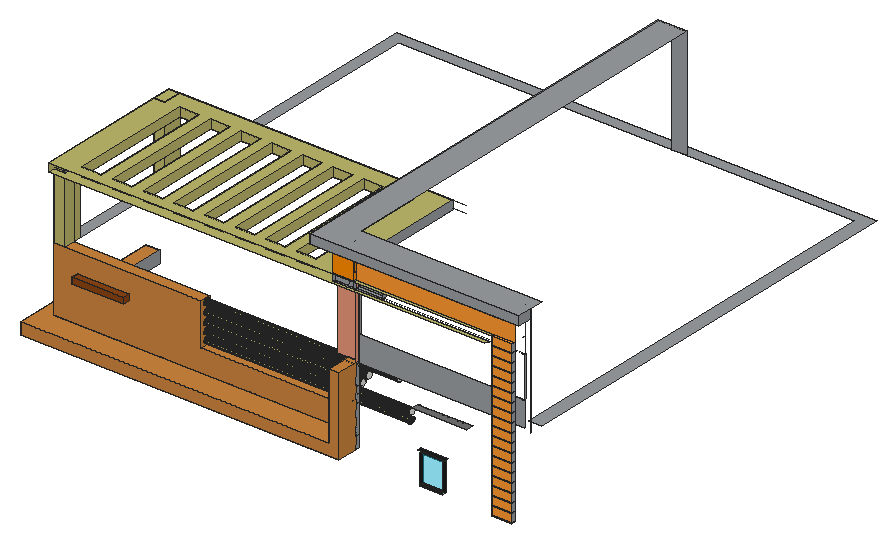
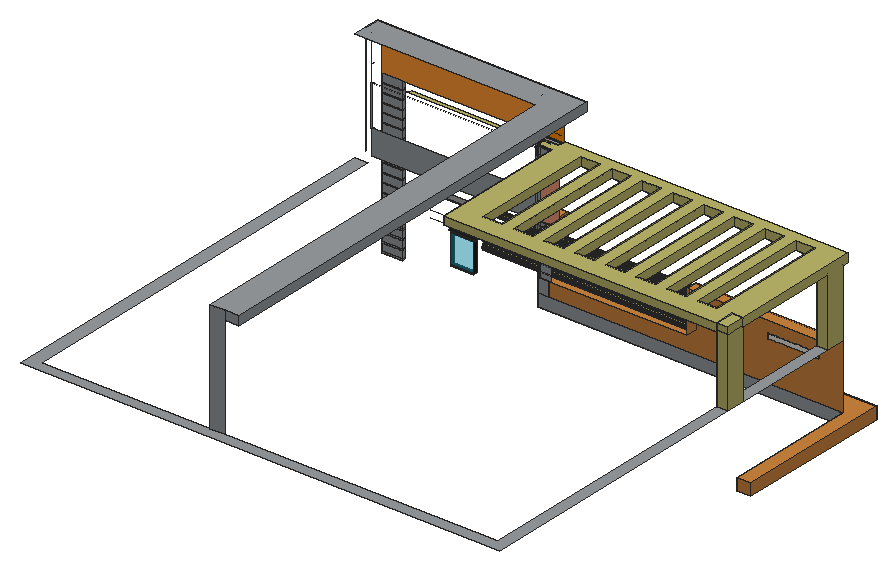
# SketchUp Ruby script. Lengths in inches.
U = 1.inch
M = Sketchup.active_model
def pt(a) = Geom::Point3d.new(a.map { |v| v * U })
def face(e, loops, mat)
  f = e.add_face(loops[0].map { |a| pt(a) })
  loops[1..].each { |l| e.add_face(l.map { |a| pt(a) }).erase! }
  f.material = f.back_material = mat if mat
  f
end
# faces: each face lists its corners as indices into pts; further lists are holes
def faces(e, pts, list, mat = nil) = list.each { |f| face(e, (f[0].is_a?(Array) ? f : [f]).map { |l| l.map { |i| pts[i] } }, mat) }
# xy, xz, yz: faces in a plane at the given z, y or x. An outline is a flat list of corners, or four numbers for a rectangle; further outlines are holes
def ring(l) = l.size == 4 ? [[l[0], l[1]], [l[2], l[1]], [l[2], l[3]], [l[0], l[3]]] : l.each_slice(2).to_a
def flat(e, list, mat, &to3) = list.each { |f| face(e, (f[0].is_a?(Array) ? f : [f]).map { |l| ring(l).map { |u, v| to3.(u, v) } }, mat) }
def xy(e, z, list, mat = nil) = flat(e, list, mat) { |x, y| [x, y, z] }
def xz(e, y, list, mat = nil) = flat(e, list, mat) { |x, z| [x, y, z] }
def yz(e, x, list, mat = nil) = flat(e, list, mat) { |y, z| [x, y, z] }
def lines(e, pts, list) = list.each { |a, b| e.add_line(pt(pts[a]), pt(pts[b])) }
# prism: a flat outline (further loops are holes) pulled along v
def prism(e, loops, v, mat = nil)
  f = face(e, loops, mat); d = Geom::Vector3d.new(v.map { |x| x * U })
  f.pushpull(f.normal.samedirection?(d) ? d.length : -d.length)
end
def box(e, o, s, mat = nil) = prism(e, [[o, [o[0] + s[0], o[1], o[2]], [o[0] + s[0], o[1] + s[1], o[2]], [o[0], o[1] + s[1], o[2]]]], [0, 0, s[2]], mat)
def at(x, y, z, deg = 0) = Geom::Transformation.translation(pt([x, y, z])) * Geom::Transformation.rotation(ORIGIN, Z_AXIS, deg.degrees)
def axes(o, x, y, z) = Geom::Transformation.new([*x, 0, *y, 0, *z, 0, *pt(o).to_a, 1])
def part(name) = M.definitions.add(name)
# library, detail: a bought-in or finely detailed component or shape, given as its bounding box
def library(name, o, s) = part(name).tap { |d| box(d.entities, o, s) }
def detail(e, o, s) = box(e.add_group.entities, o, s)
def put(e, d, t, mat = nil) = e.add_instance(d, t).tap { |i| i.material = mat if mat }
def group(e, t, mat = nil) = e.add_group.tap { |g| g.transformation = t; g.material = mat if mat }.entities
root = M.entities
M.materials.add("[0014_DarkSalmon]").color = [233, 150, 122]
M.materials.add("[0039_DarkOrange]").color = [255, 140, 0]
M.materials.add("[0040_Peru]").color = [205, 133, 63]
M.materials.add("[0043_SaddleBrown]").color = [139, 69, 19]
M.materials.add("[0057_DarkKhaki]").color = [189, 183, 107]
M.materials.add("[Color C04]").color = [255, 153, 50]
M.materials.add("[Color M05]").color = [114, 114, 114]
M.materials.add("[Color M08]").color = [30, 30, 30]
M.materials.add("[Metal Rough]").color = [153, 157, 160]
M.materials.add("[Translucent Glass Tinted]").color = [8, 201, 241]
M.materials["[Translucent Glass Tinted]"].alpha = 0.48
xy(root,144.5,[[415.14,37.17,432.3,40.17]],"[Color C04]")
xy(root,145.41,[[415.14,37.17,432.3,40.17]],"[Color C04]")
xy(root,150.37,[[359.96,31.17,379.6,34.17]],"[Color M08]")
xy(root,151.38,[[359.96,31.17,379.6,34.17]],"[Color M08]")
xy(root,152,[[415.14,37.17,432.3,40.17]],"[Color C04]")
xy(root,152.08,[[31.17,22.73,31.17,154.25,43.17,154.25,43.17,40.17,298.9,40.17,298.9,22.73]],"[0040_Peru]")
xy(root,152.08,[[43.17,40.17,298.9,40.42],[43.17,40.42,298.9,43.17]],"[Metal Rough]")
xy(root,152.91,[[415.14,37.17,432.3,40.17]],"[Color C04]")
xy(root,159.5,[[415.14,37.17,432.3,40.17]],"[Color C04]")
xy(root,160.41,[[415.14,37.17,432.3,40.17]],"[Color C04]")
xy(root,162,[[31.17,22.73,290.16,22.73,290.16,43.17,43.17,43.17,43.17,154.25,31.17,154.25]],"[0040_Peru]")
xy(root,167,[[415.14,37.17,432.3,40.17]],"[Color C04]")
xy(root,167.91,[[415.14,37.17,432.3,40.17]],"[Color C04]")
xy(root,174.5,[[415.14,37.17,432.3,40.17]],"[Metal Rough]")
xy(root,174.87,[[359.96,31.17,379.6,34.17]],"[Color M08]")
xy(root,175.41,[[415.14,37.17,432.3,40.17]],"[Color C04]")
xy(root,176.58,[[358.25,31.17,381.3125,34.17]],"[Color M08]")
xy(root,180.82,[[166.66,43.17,290.16,43.17,290.16,51.85,281.37,51.85,281.37,52.17,166.66,52.17]],"[0040_Peru]")
xy(root,180.82,[[281.37,51.85,290.16,52.17]],"[Metal Rough]")
xy(root,182,[[415.14,37.17,432.3,40.17]],"[Metal Rough]")
xy(root,182.91,[[415.14,37.17,432.3,40.17]],"[Color C04]")
xy(root,189.5,[[415.14,37.17,432.3,40.17]],"[Color C04]")
xy(root,190.41,[[415.14,37.17,432.3,40.17]],"[Color C04]")
xy(root,195.12,[[63.06,37.17,106.31,43.17]],"[0043_SaddleBrown]")
xy(root,197,[[415.14,37.17,432.3,40.17]],"[Color C04]")
xy(root,197.91,[[415.14,37.17,432.3,40.17]],"[Color C04]")
xy(root,200.18,[[63.06,37.17,106.31,43.17]],"[0043_SaddleBrown]")
xy(root,204.05,[[350.73,34.17,396.98,40.17]],"[Color M05]")
xy(root,204.05,[[350.73,40.17,389.11,40.42]],"[Metal Rough]")
xy(root,204.5,[[415.14,37.17,432.3,40.17]],"[Color C04]")
xy(root,205.41,[[415.14,37.17,432.3,40.17]],"[Color C04]")
xy(root,212,[[415.14,37.17,432.3,40.17]],"[Color C04]")
xy(root,212.91,[[415.14,37.17,432.3,40.17]],"[Color C04]")
xy(root,216.1875,[[52.23,43.17,166.66,52.17]],"[0040_Peru]")
xy(root,216.1875,[[43.17,43.17,43.17,58.8,52.17,58.8,52.17,52.17,52.23,52.17,52.23,43.17],[290.16,43.17,290.35,51.85],[290.16,51.85,293.27,52.17],[434.73,52.17,445.6,52.17,445.6,403.17,43.17,403.17,43.17,163.42,52.17,163.42,52.17,394.17,434.73,394.17],[52.17,52.17,52.23,58.8],
  [43.17,58.8,52.17,147.79],[43.17,147.79,52.17,163.42],[52.17,147.79,52.23,156.79]],"[Metal Rough]")
xy(root,217.4375,[[290.16,22.73,298.9,43.17]],"[0040_Peru]")
xy(root,217.4375,[[281.37,43.17,290.16,51.85],[290.16,43.17,290.35,51.85]],"[Metal Rough]")
xy(root,219.5,[[415.14,37.17,432.3,40.17]],"[Color C04]")
xy(root,220.41,[[415.14,37.17,432.3,40.17]],"[Color C04]")
xy(root,227,[[415.14,37.17,432.3,40.17]],"[Color C04]")
xy(root,227.91,[[415.14,37.17,432.3,40.17]],"[Color C04]")
xy(root,234.5,[[415.14,37.17,432.3,40.17]],"[Color C04]")
xy(root,235.41,[[415.14,37.17,432.3,40.17]],"[Color C04]")
xy(root,237.37,[[298.9,43.17,438.67,43.29]],"[Metal Rough]")
xy(root,242,[[415.14,37.17,432.3,40.17]],"[Color C04]")
xy(root,242.91,[[415.14,37.17,432.3,40.17]],"[Metal Rough]")
xy(root,249.5,[[415.14,37.17,432.3,40.17]],"[Color C04]")
xy(root,250.41,[[415.14,37.17,432.3,40.17]],"[Color C04]")
xy(root,257,[[415.14,37.17,432.3,40.17]],"[Color C04]")
xy(root,257.91,[[415.14,37.17,432.3,40.17]],"[Metal Rough]")
xy(root,264.5,[[415.14,37.17,432.3,40.17]],"[Color C04]")
xy(root,265.41,[[415.14,37.17,432.3,40.17]],"[Metal Rough]")
xy(root,265.6875,[[290.16,51.54,293.27,51.85]],"[Metal Rough]")
xy(root,271.4375,[[298.9,43.1,438.67,43.29]],"[Metal Rough]")
xy(root,272,[[415.14,37.17,432.3,40.17]],"[Color C04]")
xy(root,272.375,[[[43.17,37.17,43.17,43.17,52.23,43.17,52.23,52.17,52.17,52.17,52.17,58.8,43.17,58.8,43.17,147.79,52.17,147.79,52.17,163.42,281.37,163.42,281.37,50.92,293.27,50.92,293.27,43.17,281.37,43.17,281.37,40.17,411.24,40.17,409.48,37.17],[64.28,46.19,80.34,148.82],[90.03,46.19,106.09,148.82],[115.78,46.19,131.84,148.82],[141.53,46.19,157.59,148.82],[167.28,46.19,183.34,148.82],[193.03,46.19,209.09,148.82],[218.78,46.19,234.84,148.82],[244.53,46.19,260.59,148.82]]],"[0057_DarkKhaki]")
xy(root,272.91,[[415.14,37.17,432.3,40.17]],"[Metal Rough]")
xy(root,273.5,[[43.17,147.79,52.17,163.42]])
xy(root,273.5,[[293.27,38.17,298.9,38.17,298.9,40.17,281.37,40.17,281.37,38.42,293.27,38.42],[281.37,40.17,321.39,43.17],[51.48,43.17,52.17,52.17],[52.17,43.17,52.23,52.17]],"[Metal Rough]")
xy(root,279.5,[[[43.17,37.17,415.14,37.17,415.14,40.17,298.9,40.17,298.9,38.48,281.37,38.48,281.37,43.17,293.27,43.17,293.27,50.92,281.37,50.92,281.37,163.42,52.17,163.42,52.17,147.79,43.17,147.79],[64.28,46.19,80.34,148.82],[90.03,46.19,106.09,148.82],[115.78,46.19,131.84,148.82],[141.53,46.19,157.59,148.82],[167.28,46.19,183.34,148.82],[193.03,46.19,209.09,148.82],[218.78,46.19,234.84,148.82],[244.53,46.19,260.59,148.82]],[43.17,147.79,52.17,163.42]],"[0057_DarkKhaki]")
xy(root,279.5,[[415.14,37.17,432.3,40.17]],"[Color C04]")
xy(root,279.5,[[281.37,38.48,293.27,40.17],[293.27,38.48,298.9,40.17],[281.37,40.17,293.27,43.17],[293.27,40.17,298.9,43.17],[298.9,40.17,321.39,43.17],
  [281.37,50.92,293.27,51.54],[281.37,51.54,293.27,52.17]],"[Metal Rough]")
xy(root,301.86,[[281.37,38.48,298.9,38.54],[281.37,38.54,298.9,40.17]])
xy(root,301.86,[[269.68,28.17,269.68,394.17,281.37,394.17,281.37,38.48,298.9,38.48,298.9,40.17,432.3,40.17,428.02,28.17]],"[Color C04]")
xy(root,301.86,[[428.02,28.17,445.6,28.17,445.6,40.17,432.3,40.17]],"[Metal Rough]")
xy(root,309.37,[[269.68,28.17,445.6,28.17,445.6,52.17,293.27,52.17,293.27,394.17,269.68,394.17]],"[Metal Rough]")
xz(root,22.73,[[31.17,152.08,298.9,152.08,298.9,217.4375,290.16,217.4375,290.16,162,31.17,162]],"[0040_Peru]")
xz(root,28.17,[[269.68,301.86,445.6,309.37]],"[Metal Rough]")
xz(root,31.17,[[359.96,150.37,379.6,151.38]],"[Color M08]")
xz(root,34.17,[[359.96,150.37,379.6,151.38]])
xz(root,34.17,[[359.96,151.38,379.6,174.87]],"[Translucent Glass Tinted]")
xz(root,37.17,[[63.06,195.12,106.31,200.18]],"[0043_SaddleBrown]")
xz(root,37.17,[[415.14,145.41,432.3,152],[415.14,152.91,432.3,159.5],[415.14,160.41,432.3,167],[415.14,167.91,432.3,174.5],[415.14,175.41,432.3,182],
  [415.14,182.91,432.3,189.5],[415.14,190.41,432.3,197],[415.14,197.91,432.3,204.5],[415.14,205.41,432.3,212],[415.14,212.91,432.3,219.5],
  [415.14,220.41,432.3,227],[415.14,227.91,432.3,234.5],[415.14,235.41,432.3,242],[415.14,242.91,432.3,249.5],[415.14,250.41,432.3,257],
  [415.14,257.91,432.3,264.5],[415.14,265.41,432.3,272],[415.14,272.91,432.3,279.5]],"[Color C04]")
xz(root,38.48,[[281.37,279.5,298.9,301.86]],"[0039_DarkOrange]")
xz(root,40.17,[[415.14,189.5,432.3,190.41],[415.14,197,432.3,197.91],[415.14,204.5,432.3,205.41],[415.14,212,432.3,212.91],[415.14,219.5,432.3,220.41],
  [415.14,227,432.3,227.91],[415.14,234.5,432.3,235.41],[415.14,249.5,432.3,250.41],[415.14,257,432.3,257.91],[415.14,264.5,432.3,265.41],
  [415.14,272,432.3,272.91],[298.9,279.5,432.3,301.86]],"[Color C04]")
xz(root,40.17,[[415.14,144.5,432.3,145.41],[415.14,145.41,432.3,152],[415.14,152,432.3,152.91],[415.14,152.91,432.3,159.5],[415.14,159.5,432.3,160.41],
  [415.14,160.41,432.3,167],[415.14,167,432.3,167.91],[415.14,167.91,432.3,174.5],[415.14,174.5,432.3,175.41],[415.14,175.41,432.3,182],
  [415.14,182,432.3,182.91],[415.14,182.91,432.3,189.5],[415.14,190.41,432.3,197],[415.14,197.91,432.3,204.5],[415.14,205.41,432.3,212],
  [415.14,212.91,432.3,219.5],[415.14,220.41,432.3,227],[415.14,227.91,432.3,234.5],[415.14,235.41,432.3,242],[415.14,242,432.3,242.91],
  [415.14,242.91,432.3,249.5],[415.14,250.41,432.3,257],[415.14,257.91,432.3,264.5],[415.14,265.41,432.3,272],[281.37,272.375,293.27,273.5],
  [293.27,272.375,298.9,273.5],[298.9,272.375,321.39,273.5],[415.14,272.91,432.3,279.5],[281.37,273.5,293.27,279.5],[293.27,273.5,298.9,279.5]],"[Metal Rough]")
xz(root,43.17,[[63.06,195.12,106.31,200.18]])
xz(root,43.17,[[281.37,217.4375,298.9,217.4375,298.9,273.5,293.27,273.5,293.27,272.375,281.37,272.375]],"[0014_DarkSalmon]")
xz(root,43.17,[[[43.17,162,290.16,162,290.16,180.82,166.66,180.82,166.66,216.1875,43.17,216.1875],[63.06,195.12,106.31,200.18]]],"[0040_Peru]")
xz(root,43.17,[[43.17,216.1875,52.23,272.375]],"[0057_DarkKhaki]")
xz(root,43.17,[[43.17,152.08,298.9,162],[290.16,162,298.9,216.1875],[290.16,216.1875,290.35,217.4375],[290.35,216.1875,298.9,217.4375],[298.9,216.1875,438.67,237.37],
  [51.48,272.375,52.17,273.5],[52.17,272.375,52.23,273.5],[281.37,272.375,293.27,273.5],[281.37,273.5,293.27,279.5],[293.27,273.5,298.9,279.5],
  [298.9,273.5,321.39,279.5]],"[Metal Rough]")
xz(root,46.19,[[64.28,272.375,80.34,279.5],[90.03,272.375,106.09,279.5],[115.78,272.375,131.84,279.5],[141.53,272.375,157.59,279.5],[167.28,272.375,183.34,279.5],
  [193.03,272.375,209.09,279.5],[218.78,272.375,234.84,279.5],[244.53,272.375,260.59,279.5]],"[0057_DarkKhaki]")
xz(root,50.92,[[281.37,272.375,293.27,279.5]],"[Metal Rough]")
xz(root,51.85,[[281.37,180.82,290.16,216.1875],[281.37,216.1875,290.16,217.4375],[290.16,216.1875,290.35,217.4375],[290.35,216.1875,293.27,216.1875,293.27,265.6875,290.16,265.6875,290.16,217.4375,290.35,217.4375],[290.16,265.6875,293.27,271.4375]],"[Metal Rough]")
xz(root,52.17,[[52.17,216.1875,52.23,272.375],[52.17,272.375,52.23,273.5]],"[Metal Rough]")
xz(root,58.8,[[43.17,216.1875,52.17,272.375]],"[0057_DarkKhaki]")
xz(root,147.79,[[43.17,272.375,52.17,273.5],[43.17,273.5,52.17,279.5]])
xz(root,147.79,[[43.17,216.1875,52.17,272.375]],"[0057_DarkKhaki]")
xz(root,148.82,[[64.28,272.375,80.34,279.5],[90.03,272.375,106.09,279.5],[115.78,272.375,131.84,279.5],[141.53,272.375,157.59,279.5],[167.28,272.375,183.34,279.5],
  [193.03,272.375,209.09,279.5],[218.78,272.375,234.84,279.5],[244.53,272.375,260.59,279.5]],"[0057_DarkKhaki]")
xz(root,154.25,[[31.17,152.08,43.17,162]],"[0040_Peru]")
xz(root,163.42,[[43.17,216.1875,52.17,273.5],[52.17,272.375,281.37,279.5],[43.17,273.5,52.17,279.5]],"[0057_DarkKhaki]")
xz(root,394.17,[[281.37,216.1875,293.27,309.37],[269.68,301.86,281.37,309.37]],"[Metal Rough]")
yz(root,31.17,[[22.73,152.08,154.25,162]],"[0040_Peru]")
yz(root,43.17,[[43.17,216.1875,43.17,272.375,37.17,272.375,37.17,279.5,147.79,279.5,147.79,272.375,58.8,272.375,58.8,216.1875],[147.79,216.1875,163.42,273.5],[147.79,273.5,163.42,279.5]],"[0057_DarkKhaki]")
yz(root,43.17,[[43.17,152.08,154.25,162]],"[Metal Rough]")
yz(root,52.17,[[147.79,272.375,163.42,273.5],[147.79,273.5,163.42,279.5]])
yz(root,52.17,[[52.17,216.1875,58.8,272.375],[147.79,216.1875,163.42,272.375]],"[0057_DarkKhaki]")
yz(root,52.17,[[52.17,272.375,58.8,273.5]],"[Metal Rough]")
yz(root,52.23,[[43.17,216.1875,52.17,272.375]],"[0057_DarkKhaki]")
yz(root,52.23,[[43.17,272.375,52.17,273.5]],"[Metal Rough]")
yz(root,63.06,[[37.17,195.12,43.17,200.18]],"[0043_SaddleBrown]")
yz(root,64.28,[[46.19,272.375,148.82,279.5]],"[0057_DarkKhaki]")
yz(root,80.34,[[46.19,272.375,148.82,279.5]],"[0057_DarkKhaki]")
yz(root,90.03,[[46.19,272.375,148.82,279.5]],"[0057_DarkKhaki]")
yz(root,106.09,[[46.19,272.375,148.82,279.5]],"[0057_DarkKhaki]")
yz(root,106.31,[[37.17,195.12,43.17,200.18]],"[0043_SaddleBrown]")
yz(root,115.78,[[46.19,272.375,148.82,279.5]],"[0057_DarkKhaki]")
yz(root,131.84,[[46.19,272.375,148.82,279.5]],"[0057_DarkKhaki]")
yz(root,141.53,[[46.19,272.375,148.82,279.5]],"[0057_DarkKhaki]")
yz(root,157.59,[[46.19,272.375,148.82,279.5]],"[0057_DarkKhaki]")
yz(root,166.66,[[47.84,196.28,47.19,196.36,46.59,196.61,46.07,197.01,45.67,197.53,45.42,198.13,45.34,198.78,45.42,199.42,45.67,200.03,46.07,200.54,46.59,200.94,47.19,201.19,47.84,201.28,48.48,201.19,49.09,200.94,49.61,200.54,50,200.03,50.25,199.42,50.34,198.78,50.25,198.13,50,197.53,49.61,197.01,49.09,196.61,48.48,196.36],[47.84,203.84,47.19,203.92,46.59,204.17,46.07,204.57,45.67,205.09,45.42,205.69,45.34,206.34,45.42,206.99,45.67,207.59,46.07,208.11,46.59,208.5,47.19,208.75,47.84,208.84,48.48,208.75,49.09,208.5,49.61,208.11,50,207.59,50.25,206.99,50.34,206.34,50.25,205.69,50,205.09,49.61,204.57,49.09,204.17,48.48,203.92],[47.84,210.9,47.19,210.99,46.59,211.24,46.07,211.63,45.67,212.15,45.42,212.75,45.34,213.4,45.42,214.05,45.67,214.65,46.07,215.17,46.59,215.57,47.19,215.82,47.84,215.9,48.48,215.82,49.09,215.57,49.61,215.17,50,214.65,50.25,214.05,50.34,213.4,50.25,212.75,50,212.15,49.61,211.63,49.09,211.24,48.48,210.99]])
yz(root,166.66,[[[43.17,180.82,52.17,216.1875],[47.84,210.9,47.19,210.99,46.59,211.24,46.07,211.63,45.67,212.15,45.42,212.75,45.34,213.4,45.42,214.05,45.67,214.65,46.07,215.17,46.59,215.57,47.19,215.82,47.84,215.9,48.48,215.82,49.09,215.57,49.61,215.17,50,214.65,50.25,214.05,50.34,213.4,50.25,212.75,50,212.15,49.61,211.63,49.09,211.24,48.48,210.99],[47.84,203.84,47.19,203.92,46.59,204.17,46.07,204.57,45.67,205.09,45.42,205.69,45.34,206.34,45.42,206.99,45.67,207.59,46.07,208.11,46.59,208.5,47.19,208.75,47.84,208.84,48.48,208.75,49.09,208.5,49.61,208.11,50,207.59,50.25,206.99,50.34,206.34,50.25,205.69,50,205.09,49.61,204.57,49.09,204.17,48.48,203.92],[47.84,196.28,47.19,196.36,46.59,196.61,46.07,197.01,45.67,197.53,45.42,198.13,45.34,198.78,45.42,199.42,45.67,200.03,46.07,200.54,46.59,200.94,47.19,201.19,47.84,201.28,48.48,201.19,49.09,200.94,49.61,200.54,50,200.03,50.25,199.42,50.34,198.78,50.25,198.13,50,197.53,49.61,197.01,49.09,196.61,48.48,196.36],[47.88,189.39,47.23,189.47,46.63,189.72,46.11,190.12,45.71,190.64,45.46,191.24,45.38,191.89,45.46,192.54,45.71,193.14,46.11,193.66,46.63,194.05,47.23,194.3,47.88,194.39,48.53,194.3,49.13,194.05,49.65,193.66,50.04,193.14,50.29,192.54,50.38,191.89,50.29,191.24,50.04,190.64,49.65,190.12,49.13,189.72,48.53,189.47]]],"[0040_Peru]")
yz(root,167.28,[[46.19,272.375,148.82,279.5]],"[0057_DarkKhaki]")
yz(root,183.34,[[46.19,272.375,148.82,279.5]],"[0057_DarkKhaki]")
yz(root,193.03,[[46.19,272.375,148.82,279.5]],"[0057_DarkKhaki]")
yz(root,209.09,[[46.19,272.375,148.82,279.5]],"[0057_DarkKhaki]")
yz(root,218.78,[[46.19,272.375,148.82,279.5]],"[0057_DarkKhaki]")
yz(root,234.84,[[46.19,272.375,148.82,279.5]],"[0057_DarkKhaki]")
yz(root,244.53,[[46.19,272.375,148.82,279.5]],"[0057_DarkKhaki]")
yz(root,260.59,[[46.19,272.375,148.82,279.5]],"[0057_DarkKhaki]")
yz(root,269.68,[[28.17,301.86,394.17,309.37]],"[Metal Rough]")
yz(root,281.37,[[40.17,272.375,43.17,273.5],[50.92,272.375,51.54,279.5],[51.54,272.375,51.85,279.5],[51.85,272.375,52.17,279.5],[52.17,272.375,163.42,279.5],
  [38.48,273.5,40.17,279.5]],"[Metal Rough]")
yz(root,290.16,[[22.73,162,43.17,217.4375],[43.17,180.82,51.85,216.1875]],"[0040_Peru]")
yz(root,290.16,[[51.85,180.82,52.17,216.1875],[43.17,216.1875,51.85,217.4375]],"[Metal Rough]")
yz(root,290.35,[[43.17,216.1875,51.85,217.4375]],"[Metal Rough]")
yz(root,293.27,[[51.85,216.1875,52.17,265.6875],[51.54,265.6875,51.85,271.4375],[51.85,265.6875,52.17,271.4375],[51.54,271.4375,51.85,273.5],[51.85,271.4375,52.17,273.5],
  [43.17,272.375,50.92,279.5],[50.92,273.5,51.54,279.5],[51.54,273.5,51.85,279.5],[51.85,273.5,52.17,279.5],[50.92,279.5,51.85,285.1875],
  [51.85,279.5,52.17,285.1875],[51.85,285.1875,52.17,285.37]],"[Metal Rough]")
yz(root,298.9,[[47.84,196.28,48.48,196.36,49.09,196.61,49.61,197.01,50,197.53,50.25,198.13,50.34,198.78,50.25,199.42,50,200.03,49.61,200.54,49.09,200.94,48.48,201.19,47.84,201.28,47.19,201.19,46.59,200.94,46.07,200.54,45.67,200.03,45.42,199.42,45.34,198.78,45.42,198.13,45.67,197.53,46.07,197.01,46.59,196.61,47.19,196.36],[38.48,285.37,38.54,301.86]])
yz(root,298.9,[[40.17,217.4375,40.17,279.5,43.1,279.5,43.1,271.4375,43.17,271.4375,43.17,217.4375]],"[0014_DarkSalmon]")
yz(root,298.9,[[38.48,279.5,40.17,285.37],[38.54,285.37,40.17,301.86]],"[0039_DarkOrange]")
yz(root,298.9,[[22.73,152.08,40.17,217.4375]],"[0040_Peru]")
yz(root,298.9,[[40.17,152.08,40.42,162],[40.42,152.08,43.17,162],[40.17,162,40.42,216.1875],[40.42,162,43.17,216.1875],[40.17,216.1875,40.42,217.4375],
  [40.42,216.1875,43.17,217.4375],[43.17,216.1875,43.29,217.4375],[43.17,217.4375,43.29,237.37],[43.17,237.37,43.29,265.6875],[43.17,265.6875,43.29,271.4375],
  [43.1,271.4375,43.17,279.5],[43.17,271.4375,43.29,285.37],[38.48,273.5,40.17,279.5],[40.17,279.5,43.1,285.37],[43.1,279.5,43.17,285.37]],"[Metal Rough]")
yz(root,304.1,[[47.84,203.84,48.48,203.92,49.09,204.17,49.61,204.57,50,205.09,50.25,205.69,50.34,206.34,50.25,206.99,50,207.59,49.61,208.11,49.09,208.5,48.48,208.75,47.84,208.84,47.19,208.75,46.59,208.5,46.07,208.11,45.67,207.59,45.42,206.99,45.34,206.34,45.42,205.69,45.67,205.09,46.07,204.57,46.59,204.17,47.19,203.92]])
yz(root,321.39,[[40.17,273.5,43.17,279.5]],"[Metal Rough]")
yz(root,330.41,[[47.84,210.9,48.48,210.99,49.09,211.24,49.61,211.63,50,212.15,50.25,212.75,50.34,213.4,50.25,214.05,50,214.65,49.61,215.17,49.09,215.57,48.48,215.82,47.84,215.9,47.19,215.82,46.59,215.57,46.07,215.17,45.67,214.65,45.42,214.05,45.34,213.4,45.42,212.75,45.67,212.15,46.07,211.63,46.59,211.24,47.19,210.99]])
yz(root,340.1,[[47.88,189.39,48.53,189.47,49.13,189.72,49.65,190.12,50.04,190.64,50.29,191.24,50.38,191.89,50.29,192.54,50.04,193.14,49.65,193.66,49.13,194.05,48.53,194.3,47.88,194.39,47.23,194.3,46.63,194.05,46.11,193.66,45.71,193.14,45.46,192.54,45.38,191.89,45.46,191.24,45.71,190.64,46.11,190.12,46.63,189.72,47.23,189.47]])
yz(root,359.96,[[31.17,150.37,34.17,151.38]])
yz(root,359.96,[[31.17,151.38,34.17,174.87]],"[Color M08]")
yz(root,379.6,[[31.17,150.37,34.17,151.38]])
yz(root,379.6,[[31.17,151.38,34.17,174.87]],"[Color M08]")
yz(root,415.14,[[37.17,189.5,40.17,190.41],[37.17,197,40.17,197.91],[37.17,219.5,40.17,220.41]],"[Color C04]")
yz(root,415.14,[[37.17,144.5,40.17,145.41],[37.17,145.41,40.17,152],[37.17,152,40.17,152.91],[37.17,152.91,40.17,159.5],[37.17,159.5,40.17,160.41],
  [37.17,160.41,40.17,167],[37.17,167,40.17,167.91],[37.17,167.91,40.17,174.5],[37.17,174.5,40.17,175.41],[37.17,175.41,40.17,182],
  [37.17,182,40.17,182.91],[37.17,182.91,40.17,189.5],[37.17,190.41,40.17,197],[37.17,197.91,40.17,204.5],[37.17,204.5,40.17,205.41],
  [37.17,205.41,40.17,212],[37.17,212,40.17,212.91],[37.17,212.91,40.17,219.5],[37.17,220.41,40.17,227],[37.17,227,40.17,227.91],
  [37.17,227.91,40.17,234.5],[37.17,234.5,40.17,235.41],[37.17,235.41,40.17,242],[37.17,242,40.17,242.91],[37.17,242.91,40.17,249.5],
  [37.17,249.5,40.17,250.41],[37.17,250.41,40.17,257],[37.17,257,40.17,257.91],[37.17,257.91,40.17,264.5],[37.17,264.5,40.17,265.41],
  [37.17,265.41,40.17,272],[37.17,272,40.17,272.91],[37.17,272.91,40.17,279.5]],"[Metal Rough]")
yz(root,432.3,[[37.17,145.41,40.17,152],[37.17,152.91,40.17,159.5],[37.17,160.41,40.17,167],[37.17,167.91,40.17,174.5],[37.17,175.41,40.17,182],
  [37.17,182.91,40.17,189.5],[37.17,190.41,40.17,197],[37.17,197.91,40.17,204.5],[37.17,205.41,40.17,212],[37.17,212.91,40.17,219.5],
  [37.17,220.41,40.17,227],[37.17,227.91,40.17,234.5],[37.17,235.41,40.17,242],[37.17,242.91,40.17,249.5],[37.17,250.41,40.17,257],
  [37.17,257.91,40.17,264.5],[37.17,265.41,40.17,272],[37.17,272.91,40.17,279.5]],"[Metal Rough]")
yz(root,438.67,[[43.17,237.37,43.85,271.4375]],"[Metal Rough]")
yz(root,445.6,[[40.17,216.1875,40.42,237.37],[40.17,237.37,40.42,285.37],[40.17,285.37,40.42,309.37],[28.17,301.86,40.17,309.37]],"[Metal Rough]")
p = [[166.66,47.23,182.79],[166.66,47.88,182.7],[340.1,47.88,182.7],[340.1,47.23,182.79],[166.66,48.53,182.79],[340.1,48.53,182.79],
  [166.66,46.63,183.04],[340.1,46.63,183.04],[166.66,49.13,183.04],[340.1,49.13,183.04],[166.66,46.11,183.43],[340.1,46.11,183.43],
  [166.66,49.65,183.43],[340.1,49.65,183.43],[166.66,45.71,183.95],[340.1,45.71,183.95],[166.66,50.04,183.95],[340.1,50.04,183.95],
  [166.66,45.46,184.55],[340.1,45.46,184.55],[166.66,50.29,184.55],[340.1,50.29,184.55],[166.66,45.38,185.2],[340.1,45.38,185.2],
  [166.66,50.38,185.2],[340.1,50.38,185.2],[166.66,45.46,185.85],[340.1,45.46,185.85],[166.66,50.29,185.85],[340.1,50.29,185.85],
  [166.66,45.71,186.45],[340.1,45.71,186.45],[166.66,50.04,186.45],[340.1,50.04,186.45],[166.66,46.11,186.97],[340.1,46.11,186.97],
  [166.66,49.65,186.97],[340.1,49.65,186.97],[166.66,46.63,187.37],[340.1,46.63,187.37],[166.66,49.13,187.37],[340.1,49.13,187.37],
  [166.66,47.23,187.62],[340.1,47.23,187.62],[166.66,48.53,187.62],[340.1,48.53,187.62],[166.66,47.88,187.7],[340.1,47.88,187.7],
  [166.66,47.23,189.47],[166.66,47.88,189.39],[340.1,47.88,189.39],[340.1,47.23,189.47],[166.66,48.53,189.47],[340.1,48.53,189.47],
  [166.66,46.63,189.72],[340.1,46.63,189.72],[166.66,49.13,189.72],[340.1,49.13,189.72],[166.66,46.11,190.12],[340.1,46.11,190.12],
  [166.66,49.65,190.12],[340.1,49.65,190.12],[166.66,45.71,190.64],[340.1,45.71,190.64],[166.66,50.04,190.64],[340.1,50.04,190.64],
  [166.66,45.46,191.24],[340.1,45.46,191.24],[166.66,50.29,191.24],[340.1,50.29,191.24],[166.66,45.38,191.89],[340.1,45.38,191.89],
  [166.66,50.38,191.89],[340.1,50.38,191.89],[166.66,45.46,192.54],[340.1,45.46,192.54],[166.66,50.29,192.54],[340.1,50.29,192.54],
  [166.66,45.71,193.14],[340.1,45.71,193.14],[166.66,50.04,193.14],[340.1,50.04,193.14],[166.66,46.11,193.66],[340.1,46.11,193.66],
  [166.66,49.65,193.66],[340.1,49.65,193.66],[166.66,46.63,194.05],[340.1,46.63,194.05],[166.66,49.13,194.05],[340.1,49.13,194.05],
  [166.66,47.23,194.3],[340.1,47.23,194.3],[166.66,48.53,194.3],[340.1,48.53,194.3],[166.66,47.88,194.39],[340.1,47.88,194.39],
  [166.66,47.19,196.36],[166.66,47.84,196.28],[298.9,47.84,196.28],[298.9,47.19,196.36],[166.66,48.48,196.36],[298.9,48.48,196.36],
  [166.66,46.59,196.61],[298.9,46.59,196.61],[166.66,49.09,196.61],[298.9,49.09,196.61],[166.66,46.07,197.01],[298.9,46.07,197.01],
  [166.66,49.61,197.01],[298.9,49.61,197.01],[166.66,45.67,197.53],[298.9,45.67,197.53],[166.66,50,197.53],[298.9,50,197.53],
  [166.66,45.42,198.13],[298.9,45.42,198.13],[166.66,50.25,198.13],[298.9,50.25,198.13],[166.66,45.34,198.78],[298.9,45.34,198.78],
  [166.66,50.34,198.78],[298.9,50.34,198.78],[166.66,45.42,199.42],[298.9,45.42,199.42],[166.66,50.25,199.42],[298.9,50.25,199.42],
  [166.66,45.67,200.03],[298.9,45.67,200.03],[166.66,50,200.03],[298.9,50,200.03],[166.66,46.07,200.54],[298.9,46.07,200.54],
  [166.66,49.61,200.54],[298.9,49.61,200.54],[166.66,46.59,200.94],[298.9,46.59,200.94],[166.66,49.09,200.94],[298.9,49.09,200.94],
  [166.66,47.19,201.19],[298.9,47.19,201.19],[166.66,48.48,201.19],[298.9,48.48,201.19],[166.66,47.84,201.28],[298.9,47.84,201.28],
  [166.66,47.19,203.92],[166.66,47.84,203.84],[304.1,47.84,203.84],[304.1,47.19,203.92],[166.66,48.48,203.92],[304.1,48.48,203.92],
  [166.66,46.59,204.17],[304.1,46.59,204.17],[166.66,49.09,204.17],[304.1,49.09,204.17],[166.66,46.07,204.57],[304.1,46.07,204.57],
  [166.66,49.61,204.57],[304.1,49.61,204.57],[166.66,45.67,205.09],[304.1,45.67,205.09],[166.66,50,205.09],[304.1,50,205.09],
  [166.66,45.42,205.69],[304.1,45.42,205.69],[166.66,50.25,205.69],[304.1,50.25,205.69],[166.66,45.34,206.34],[304.1,45.34,206.34],
  [166.66,50.34,206.34],[304.1,50.34,206.34],[166.66,45.42,206.99],[304.1,45.42,206.99],[166.66,50.25,206.99],[304.1,50.25,206.99],
  [166.66,45.67,207.59],[304.1,45.67,207.59],[166.66,50,207.59],[304.1,50,207.59],[166.66,46.07,208.11],[304.1,46.07,208.11],
  [166.66,49.61,208.11],[304.1,49.61,208.11],[166.66,46.59,208.5],[304.1,46.59,208.5],[166.66,49.09,208.5],[304.1,49.09,208.5],
  [166.66,47.19,208.75],[304.1,47.19,208.75],[166.66,48.48,208.75],[304.1,48.48,208.75],[166.66,47.84,208.84],[304.1,47.84,208.84],
  [166.66,47.19,210.99],[166.66,47.84,210.9],[330.41,47.84,210.9],[330.41,47.19,210.99],[166.66,48.48,210.99],[330.41,48.48,210.99],
  [166.66,46.59,211.24],[330.41,46.59,211.24],[166.66,49.09,211.24],[330.41,49.09,211.24],[166.66,46.07,211.63],[330.41,46.07,211.63],
  [166.66,49.61,211.63],[330.41,49.61,211.63],[166.66,45.67,212.15],[330.41,45.67,212.15],[166.66,50,212.15],[330.41,50,212.15],
  [166.66,45.42,212.75],[330.41,45.42,212.75],[166.66,50.25,212.75],[330.41,50.25,212.75],[166.66,45.34,213.4],[330.41,45.34,213.4],
  [166.66,50.34,213.4],[330.41,50.34,213.4],[166.66,45.42,214.05],[330.41,45.42,214.05],[166.66,50.25,214.05],[330.41,50.25,214.05],
  [166.66,45.67,214.65],[330.41,45.67,214.65],[166.66,50,214.65],[330.41,50,214.65],[166.66,46.07,215.17],[330.41,46.07,215.17],
  [166.66,49.61,215.17],[330.41,49.61,215.17],[166.66,46.59,215.57],[330.41,46.59,215.57],[166.66,49.09,215.57],[330.41,49.09,215.57],
  [166.66,47.19,215.82],[330.41,47.19,215.82],[166.66,48.48,215.82],[330.41,48.48,215.82],[166.66,47.84,215.9],[330.41,47.84,215.9],
  [281.37,163.42,279.5],[293.27,163.42,279.5],[290.16,43.17,271.4375],[290.16,51.85,271.4375],[290.16,43.17,285.1875],[290.16,51.85,285.1875],
  [290.16,43.17,284.3],[290.16,51.85,284.3],[281.37,51.85,284.3],[290.16,51.85,285.37],[293.27,50.92,285.1875],[293.27,50.92,285.37],
  [290.16,51.54,265.6875],[281.37,51.54,265.6875],[281.37,163.42,273.5],[293.27,163.42,273.5],[438.67,43.1,271.4375],[438.67,43.1,285.37],
  [438.67,40.42,285.37],[51.48,43.17,273.5],[43.17,43.17,273.5],[52.17,58.8,273.5],[43.17,58.8,273.5],[438.67,43.1,309.37],
  [298.9,40.17,301.86],[298.9,40.17,309.37],[298.9,38.48,301.86],[298.9,38.48,309.37],[298.9,38.17,273.5],[298.9,38.17,272.375],
  [298.9,40.17,285.37],[281.37,40.17,285.37]]
faces(root,p,[[0,1,2,3],[1,4,5,2],[6,0,3,7],[4,8,9,5],[10,6,7,11],[8,12,13,9],[14,10,11,15],[12,16,17,13],
  [18,14,15,19],[16,20,21,17],[22,18,19,23],[20,24,25,21],[26,22,23,27],[24,28,29,25],[30,26,27,31],[28,32,33,29],
  [34,30,31,35],[32,36,37,33],[38,34,35,39],[36,40,41,37],[42,38,39,43],[40,44,45,41],[46,42,43,47],[44,46,47,45],
  [48,49,50,51],[49,52,53,50],[54,48,51,55],[52,56,57,53],[58,54,55,59],[56,60,61,57],[62,58,59,63],[60,64,65,61],
  [66,62,63,67],[64,68,69,65],[70,66,67,71],[68,72,73,69],[74,70,71,75],[72,76,77,73],[78,74,75,79],[76,80,81,77],
  [82,78,79,83],[80,84,85,81],[86,82,83,87],[84,88,89,85],[90,86,87,91],[88,92,93,89],[94,90,91,95],[92,94,95,93],
  [96,97,98,99],[97,100,101,98],[102,96,99,103],[100,104,105,101],[106,102,103,107],[104,108,109,105],[110,106,107,111],[108,112,113,109],
  [114,110,111,115],[112,116,117,113],[118,114,115,119],[116,120,121,117],[122,118,119,123],[120,124,125,121],[126,122,123,127],[124,128,129,125],
  [130,126,127,131],[128,132,133,129],[134,130,131,135],[132,136,137,133],[138,134,135,139],[136,140,141,137],[142,138,139,143],[140,142,143,141],
  [144,145,146,147],[145,148,149,146],[150,144,147,151],[148,152,153,149],[154,150,151,155],[152,156,157,153],[158,154,155,159],[156,160,161,157],
  [162,158,159,163],[160,164,165,161],[166,162,163,167],[164,168,169,165],[170,166,167,171],[168,172,173,169],[174,170,171,175],[172,176,177,173],
  [178,174,175,179],[176,180,181,177],[182,178,179,183],[180,184,185,181],[186,182,183,187],[184,188,189,185],[190,186,187,191],[188,190,191,189],
  [192,193,194,195],[193,196,197,194],[198,192,195,199],[196,200,201,197],[202,198,199,203],[200,204,205,201],[206,202,203,207],[204,208,209,205],
  [210,206,207,211],[208,212,213,209],[214,210,211,215],[212,216,217,213],[218,214,215,219],[216,220,221,217],[222,218,219,223],[220,224,225,221],
  [226,222,223,227],[224,228,229,225],[230,226,227,231],[228,232,233,229],[234,230,231,235],[232,236,237,233],[238,234,235,239],[236,238,239,237]],"[0057_DarkKhaki]")
lines(root,p,[[240,241],[242,243],[244,245],[246,247],[247,248],[243,247],[247,245],[245,249],[250,251],[252,253],[254,255],[256,257],
  [257,258],[259,260],[261,262],[257,263],[264,265],[266,267],[268,269],[270,271]])
